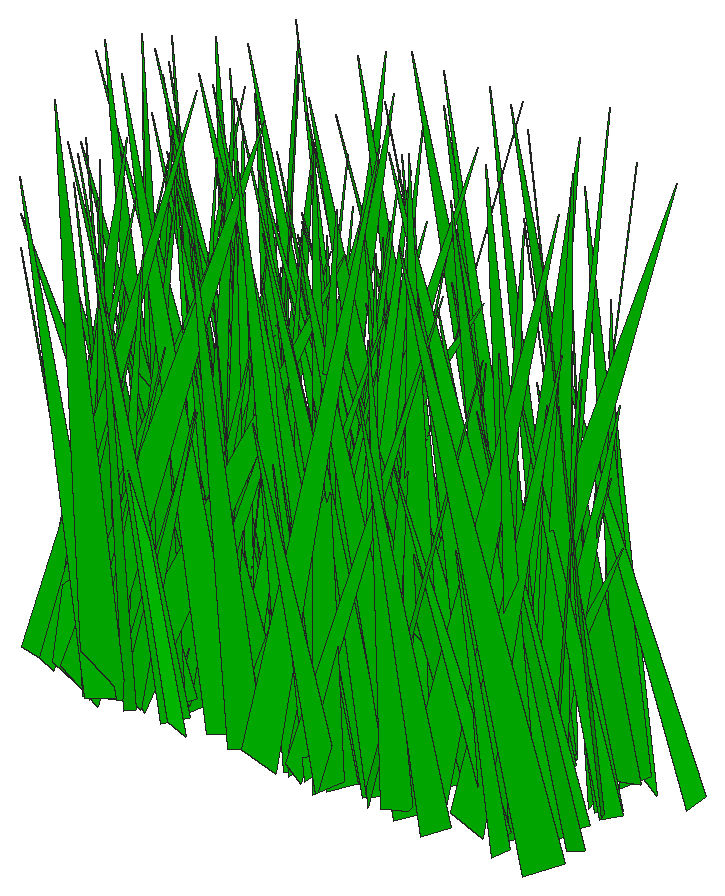
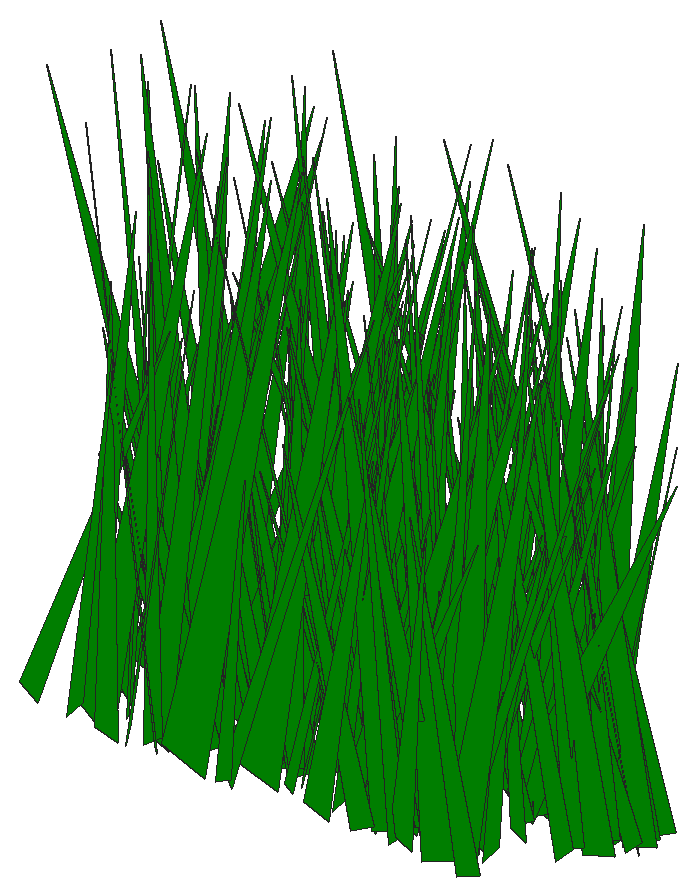
# SketchUp Ruby script. Lengths in inches.
U = 1.inch
M = Sketchup.active_model
def pt(a) = Geom::Point3d.new(a.map { |v| v * U })
def face(e, loops, mat)
  f = e.add_face(loops[0].map { |a| pt(a) })
  loops[1..].each { |l| e.add_face(l.map { |a| pt(a) }).erase! }
  f.material = f.back_material = mat if mat
  f
end
# faces: each face lists its corners as indices into pts; further lists are holes
def faces(e, pts, list, mat = nil) = list.each { |f| face(e, (f[0].is_a?(Array) ? f : [f]).map { |l| l.map { |i| pts[i] } }, mat) }
# xy, xz, yz: faces in a plane at the given z, y or x. An outline is a flat list of corners, or four numbers for a rectangle; further outlines are holes
def ring(l) = l.size == 4 ? [[l[0], l[1]], [l[2], l[1]], [l[2], l[3]], [l[0], l[3]]] : l.each_slice(2).to_a
def flat(e, list, mat, &to3) = list.each { |f| face(e, (f[0].is_a?(Array) ? f : [f]).map { |l| ring(l).map { |u, v| to3.(u, v) } }, mat) }
def xy(e, z, list, mat = nil) = flat(e, list, mat) { |x, y| [x, y, z] }
def xz(e, y, list, mat = nil) = flat(e, list, mat) { |x, z| [x, y, z] }
def yz(e, x, list, mat = nil) = flat(e, list, mat) { |y, z| [x, y, z] }
def lines(e, pts, list) = list.each { |a, b| e.add_line(pt(pts[a]), pt(pts[b])) }
# prism: a flat outline (further loops are holes) pulled along v
def prism(e, loops, v, mat = nil)
  f = face(e, loops, mat); d = Geom::Vector3d.new(v.map { |x| x * U })
  f.pushpull(f.normal.samedirection?(d) ? d.length : -d.length)
end
def box(e, o, s, mat = nil) = prism(e, [[o, [o[0] + s[0], o[1], o[2]], [o[0] + s[0], o[1] + s[1], o[2]], [o[0], o[1] + s[1], o[2]]]], [0, 0, s[2]], mat)
def at(x, y, z, deg = 0) = Geom::Transformation.translation(pt([x, y, z])) * Geom::Transformation.rotation(ORIGIN, Z_AXIS, deg.degrees)
def axes(o, x, y, z) = Geom::Transformation.new([*x, 0, *y, 0, *z, 0, *pt(o).to_a, 1])
def part(name) = M.definitions.add(name)
# library, detail: a bought-in or finely detailed component or shape, given as its bounding box
def library(name, o, s) = part(name).tap { |d| box(d.entities, o, s) }
def detail(e, o, s) = box(e.add_group.entities, o, s)
def put(e, d, t, mat = nil) = e.add_instance(d, t).tap { |i| i.material = mat if mat }
def group(e, t, mat = nil) = e.add_group.tap { |g| g.transformation = t; g.material = mat if mat }.entities
root = M.entities
M.materials.add("[Color G06]").color = [0, 204, 0]
c1 = part("fur_instance\#9")
p = [[0.8125,0,1.79],[0.67,-0.02,1.48],[0,-0.11,0],[0,0.11,0]]
faces(c1.entities,p,[[0,1,2,3]])
put(root,c1,axes([80.09,16.16,4.28],[-3.96504,0.00462,0.61887],[-0.1065,0.52435,-1.97341],[0.40152,0.18466,5.58803]),"[Color G06]")
put(root,c1,axes([81.36,17.7,4.28],[-2.4045,0.50598,0.05745],[3.24631,0.29707,2.94108],[-1.62149,-0.15557,5.80301]),"[Color G06]")
put(root,c1,axes([77.95,17.43,4.28],[1.58448,-0.59409,2.33966],[-4.52208,-0.18675,1.39339],[0.39011,0.24818,6.64912]),"[Color G06]")
put(root,c1,axes([81.13,20.35,4.28],[-5.10358,0.12595,0.06674],[0.89659,0.70004,1.38494],[-0.11823,-0.12831,7.62141]),"[Color G06]")
put(root,c1,axes([78.5,17.36,4.28],[-2.23107,0.3733,1.08265],[2.29187,0.32118,-2.17174],[1.56163,0.06197,4.73401]),"[Color G06]")
put(root,c1,axes([80.28,15.98,4.28],[-2.39441,0.52902,0.87524],[3.82716,0.32155,1.06103],[-0.29682,-0.12147,6.6204]),"[Color G06]")
put(root,c1,axes([79.65,17.76,4.28],[-4.27684,-0.24388,1.66183],[-1.50261,0.60978,1.64164],[1.4273,-0.08881,6.70788]),"[Color G06]")
put(root,c1,axes([77.92,16.99,4.28],[3.84261,0.30678,1.26542],[2.34016,-0.52363,-1.29043],[-0.2839,-0.16391,6.49069]),"[Color G06]")
put(root,c1,axes([78.72,17.62,4.28],[1.63511,0.35667,2.41092],[3.02113,-0.2038,-1.11332],[-0.13155,-0.24709,4.39848]),"[Color G06]")
put(root,c1,axes([78.9,16.41,4.28],[-1.91184,0.4234,1.31875],[2.85671,0.29293,-1.5526],[1.35528,-0.02017,5.13294]),"[Color G06]")
put(root,c1,axes([78.42,17.22,4.28],[3.46241,0.21076,0.30932],[1.42342,-0.47208,1.36022],[-0.54874,0.10528,5.48009]),"[Color G06]")
put(root,c1,axes([78.36,16.45,4.28],[2.42093,-0.21005,0.71566],[-1.58046,-0.31995,1.15486],[0.02258,0.12672,4.10204]),"[Color G06]")
put(root,c1,axes([78.46,18.35,4.28],[0.43266,0.63211,0.99472],[4.49647,-0.0407,-1.39792],[0.8791,-0.10294,6.66058]),"[Color G06]")
put(root,c1,axes([78.11,17.37,4.28],[4.86594,0.18567,0.54154],[1.17861,-0.65553,2.16249],[-0.71768,0.18233,7.2231]),"[Color G06]")
put(root,c1,axes([79.97,17.38,4.28],[-4.23289,-0.34339,0.66218],[-2.11478,0.5559,2.9186],[1.33719,-0.20785,6.71195]),"[Color G06]")
put(root,c1,axes([81.48,17.78,4.28],[-4.50555,-0.20228,0.60661],[-1.50622,0.60311,-1.8868],[-0.01596,0.1849,6.81801]),"[Color G06]")
put(root,c1,axes([80.9,20.61,4.28],[0.2752,-0.65623,1.88496],[-4.66441,-0.08636,-1.93271],[-1.40715,0.15794,6.77517]),"[Color G06]")
put(root,c1,axes([79.14,18.41,4.28],[3.6223,0.36259,2.56895],[2.99852,-0.5057,-1.24506],[-0.85112,-0.23845,6.54687]),"[Color G06]")
put(root,c1,axes([79.79,16.81,4.28],[-3.23329,-0.49254,1.52623],[-3.33124,0.47268,1.75922],[1.55612,-0.01151,6.93722]),"[Color G06]")
put(root,c1,axes([80.375,16.03,4.28],[0.81309,-0.78469,0.50058],[-5.56406,-0.11929,-1.29318],[-0.90518,0.0284,8.3987]),"[Color G06]")
put(root,c1,axes([81.125,19.6875,4.28],[-0.21231,0.4211,1.68724],[3.02032,-0.0292,1.68604],[-1.12756,-0.1575,4.19858]),"[Color G06]")
put(root,c1,axes([81.89,16.99,4.28],[-2.15082,0.47994,0.40651],[3.29774,0.27236,2.03593],[-1.02201,-0.13119,5.71389]),"[Color G06]")
put(root,c1,axes([80.46,19.91,4.28],[-4.83651,-0.45011,1.24887],[-2.8033,0.66008,3.07866],[1.80518,-0.18089,8.12692]),"[Color G06]")
put(root,c1,axes([81.21,17.43,4.28],[0.82147,0.73645,2.48814],[5.30748,-0.17164,1.92187],[-1.57919,-0.19378,7.7535]),"[Color G06]")
put(root,c1,axes([77.89,16.61,4.28],[5.38802,-0.39803,0.24516],[-2.84975,-0.7437,1.1956],[0.23092,0.10922,9.03424]),"[Color G06]")
put(root,c1,axes([80.7,17.61,4.28],[-4.16965,0.39593,1.84315],[2.72244,0.60634,-1.20494],[1.47337,0.00011,7.44256]),"[Color G06]")
put(root,c1,axes([81.95,19,4.28],[-2.47231,0.30424,0.98661],[2.19111,0.27974,2.35509],[-0.62856,-0.22153,4.329]),"[Color G06]")
put(root,c1,axes([78.05,17.54,4.28],[4.01317,0.37829,0.17792],[2.59468,-0.52549,-2.38462],[0.80068,-0.19316,6.83579]),"[Color G06]")
put(root,c1,axes([79.08,18.86,4.28],[5.07893,-0.20615,1.62963],[-1.70837,-0.69439,1.80264],[-0.67517,0.20626,7.6976]),"[Color G06]")
put(root,c1,axes([81.15,15.97,4.28],[3.31982,0.29513,2.99147],[2.00912,-0.5384,1.12136],[-2.10928,-0.04832,5.77642]),"[Color G06]")
put(root,c1,axes([82.82,17.6,4.28],[-2.6484,-0.58234,1.01179],[-4.0563,0.31788,-2.69933],[-1.20194,0.21035,6.88023]),"[Color G06]")
put(root,c1,axes([80.11,16.8,4.28],[3.64205,-0.35592,0.44862],[-2.36631,-0.49274,-1.99603],[-1.00267,-0.12994,6.34016]),"[Color G06]")
put(root,c1,axes([81.54,19.76,4.28],[0.99429,0.79231,0.0814],[5.53838,-0.13686,1.91316],[-1.27012,0.02348,8.40609]),"[Color G06]")
put(root,c1,axes([79.84,16.05,4.28],[3.50765,-0.04486,0.99817],[-0.56639,-0.45277,2.10829],[-0.47827,0.20717,4.82385]),"[Color G06]")
put(root,c1,axes([82.6,17.38,4.28],[-3.57372,-0.17571,0.20364],[-1.24049,0.47327,-1.71721],[-0.25986,0.15722,5.39686]),"[Color G06]")
put(root,c1,axes([82.54,15.93,4.28],[-4.81615,0.25556,0.10319],[1.78872,0.66051,-1.43588],[0.40512,0.12186,7.56662]),"[Color G06]")
put(root,c1,axes([80.23,16.99,4.28],[3.20722,0.40339,2.50922],[3.29254,-0.43784,-1.31478],[-0.58841,-0.25125,6.3199]),"[Color G06]")
put(root,c1,axes([78.59,16.93,4.28],[2.98606,-0.61165,0.26624],[-4.16026,-0.3847,2.70231],[1.40121,0.16127,7.45594]),"[Color G06]")
put(root,c1,axes([81.77,16.75,4.28],[4.04095,0.57837,2.58795],[3.68795,-0.61227,2.85567],[-2.5691,0.0308,8.16993]),"[Color G06]")
put(root,c1,axes([80.54,18.77,4.28],[4.36803,-0.24739,1.48073],[-1.54639,-0.61719,-1.65582],[-1.31822,-0.09573,6.84895]),"[Color G06]")
put(root,c1,axes([82.59,18.78,4.28],[-1.58143,0.40161,0.24801],[2.74135,0.20099,1.65805],[-0.89849,-0.09364,4.6223]),"[Color G06]")
put(root,c1,axes([82.26,16.23,4.28],[0.70188,-0.54769,1.43807],[-3.75426,-0.13886,-1.9821],[-1.50258,0.09111,5.6241]),"[Color G06]")
put(root,c1,axes([80.24,21.03,4.28],[1.16188,-0.42472,0.47893],[-3.01179,-0.14979,1.06163],[0.5554,0.07622,4.75501]),"[Color G06]")
put(root,c1,axes([81.04,19.32,4.28],[2.43605,-0.25594,0.32134],[-1.63588,-0.32174,-1.73621],[-0.85956,-0.11302,4.21501]),"[Color G06]")
put(root,c1,axes([83.5,19.28,4.28],[-4.86937,0.36862,1.36795],[2.79614,0.63358,2.62044],[-0.08479,-0.27555,7.85534]),"[Color G06]")
put(root,c1,axes([81.9,20.03,4.28],[-4.57528,0.18823,3.13164],[1.9138,0.65659,1.71217],[1.59683,-0.24761,6.92083]),"[Color G06]")
put(root,c1,axes([83.37,18.5,4.28],[-4.60442,0.28891,0.86362],[2.1486,0.62669,1.50444],[0.10062,-0.16124,7.39477]),"[Color G06]")
put(root,c1,axes([80.6,16.57,4.28],[0.32697,-0.38482,1.37835],[-2.73268,0.00383,1.57089],[0.99929,0.13639,3.8448]),"[Color G06]")
put(root,c1,axes([82.48,17.54,4.28],[-0.30271,0.39217,0.95163],[2.805,0.01935,1.07699],[-0.6685,-0.09639,4.0881]),"[Color G06]")
put(root,c1,axes([82.28,19.53,4.28],[0.708,-0.5248,0.93803],[-3.7172,-0.11495,-1.12057],[-0.86046,0.06476,5.61274]),"[Color G06]")
put(root,c1,axes([82.01,19.58,4.28],[-2.39476,-0.4155,0.18423],[-2.85308,0.32562,1.52115],[0.86817,-0.07604,5.50717]),"[Color G06]")
put(root,c1,axes([80.94,16.3125,4.28],[1.54694,0.33616,0.96474],[2.47753,-0.19414,-1.10306],[0.29989,-0.13017,4.13641]),"[Color G06]")
put(root,c1,axes([83.54,16.49,4.28],[-2.62366,0.70015,1.24289],[5.05123,0.3423,1.66728],[-0.62171,-0.17358,8.30114]),"[Color G06]")
put(root,c1,axes([83.1,19.95,4.28],[0.71881,-0.58378,0.80663],[-3.92306,-0.12057,-2.21494],[-1.55795,0.03426,5.94958]),"[Color G06]")
put(root,c1,axes([82.52,20.74,4.28],[0.67687,0.44536,0.3364],[3.07735,-0.09935,1.27806],[-0.88357,-0.00485,4.70898]),"[Color G06]")
put(root,c1,axes([80.77,18.22,4.28],[2.3137,0.35161,0.89932],[2.56104,-0.29262,-1.57519],[0.40143,-0.15971,4.86608]),"[Color G06]")
put(root,c1,axes([81.23,20.91,4.28],[-0.73264,-0.68843,0.33457],[-4.769,0.10676,1.9084],[1.29609,0.00369,7.21113]),"[Color G06]")
put(root,c1,axes([81.78,19.58,4.28],[3.83466,-0.10946,2.37796],[-1.12493,-0.5586,1.09833],[-1.37193,0.15207,5.74599]),"[Color G06]")
put(root,c1,axes([83.74,17.68,4.28],[-5.72432,-0.07873,1.63527],[-0.93594,0.74967,-3.1724],[0.79994,0.31376,7.99019]),"[Color G06]")
put(root,c1,axes([79.58,16.12,4.28],[3.16824,0.74272,0.60226],[5.15125,-0.40757,-2.7925],[1.41278,-0.17952,8.83135]),"[Color G06]")
put(root,c1,axes([83.78,20.46,4.28],[-1.65602,-0.40717,0.43226],[-2.72838,0.19664,-2.07052],[-1.07954,0.12761,4.56983]),"[Color G06]")
put(root,c1,axes([84.27,19.66,4.28],[-3.87879,0.52171,0.42569],[3.70429,0.52334,1.71482],[-0.59736,-0.14226,7.86975]),"[Color G06]")
put(root,c1,axes([83.77,17.71,4.28],[-0.12418,-0.69923,0.11328],[-4.71267,0.01266,-2.56608],[-1.71484,0.01586,7.04383]),"[Color G06]")
put(root,c1,axes([82.5,18.28,4.28],[-3.40951,0.52314,1.3132],[3.59675,0.49079,-1.60056],[1.38195,0.01331,7.40564]),"[Color G06]")
put(root,c1,axes([83.08,16.58,4.28],[-4.76756,0.23054,1.68564],[1.47211,0.67923,-1.37104],[1.3558,0.07317,7.41606]),"[Color G06]")
put(root,c1,axes([82.35,17.15,4.28],[4.03013,0.64486,0.15163],[4.28978,-0.52808,3.3066],[-1.73031,0.19277,8.55088]),"[Color G06]")
put(root,c1,axes([82.41,19.34,4.28],[4.96519,0.45977,1.55514],[2.76899,-0.68085,3.37523],[-2.07035,0.19203,8.24378]),"[Color G06]")
put(root,c1,axes([81.57,17.21,4.28],[-0.53189,-0.41062,2.41143],[-3.05598,0.15358,1.49841],[1.3911,0.18038,4.21372]),"[Color G06]")
put(root,c1,axes([81.42,20.64,4.28],[0.81439,0.59826,0.36984],[4.18237,-0.10227,-1.5681],[0.98764,-0.06024,6.33544]),"[Color G06]")
put(root,c1,axes([83.79,19.01,4.28],[-4.3787,-0.31758,0.36115],[-2.15416,0.5958,1.84404],[0.77758,-0.13777,7.14234]),"[Color G06]")
put(root,c1,axes([82.88,17.54,4.28],[1.86528,0.58077,0.34705],[4.04047,-0.26037,1.54429],[-1.03668,0.03018,6.64334]),"[Color G06]")
put(root,c1,axes([85.39,18.63,4.28],[-4.17033,0.42514,0.08923],[2.86207,0.54084,2.7787],[-1.05236,-0.21389,7.20354]),"[Color G06]")
put(root,c1,axes([83.98,19.09,4.28],[1.74604,0.75305,0.44387],[4.99882,-0.24131,3.10552],[-2.06482,0.05259,7.89364]),"[Color G06]")
put(root,c1,axes([82.45,18.3,4.28],[3.80681,0.12833,1.46285],[0.57715,-0.52655,1.95156],[-1.21321,0.15219,5.51854]),"[Color G06]")
put(root,c1,axes([83.26,19.1875,4.28],[1.87152,-0.72948,0.52679],[-5.11595,-0.26549,-1.63416],[-1.14797,-0.00609,8.14147]),"[Color G06]")
put(root,c1,axes([82.64,20.72,4.28],[3.48071,-0.19732,2.6462],[-1.99959,-0.48037,1.76035],[-1.06715,0.25649,5.33259]),"[Color G06]")
put(root,c1,axes([83.52,17.32,4.28],[-3.46008,-0.14982,1.3927],[-0.8941,0.49495,1.15466],[1.10601,-0.06859,5.29038]),"[Color G06]")
put(root,c1,axes([82.79,18.76,4.28],[5.25675,0.11325,2.77653],[0.2932,-0.75477,2.29663],[-2.0062,0.18644,7.61086]),"[Color G06]")
put(root,c1,axes([82.74,17.22,4.28],[3.57711,0.39826,0.4126],[2.65145,-0.48231,2.13218],[-1.09673,0.13292,6.5005]),"[Color G06]")
put(root,c1,axes([84.54,20.16,4.28],[-2.0182,-0.34557,0.81583],[-2.49557,0.25267,-1.49552],[-0.45975,0.14544,4.5365]),"[Color G06]")
put(root,c1,axes([84.72,20.3,4.28],[-5.59106,0.18018,1.37785],[1.1167,0.78103,-1.61102],[1.12807,0.1199,8.42385]),"[Color G06]")
put(root,c1,axes([83.03,19.55,4.28],[4.8492,0.30832,1.14131],[1.64095,-0.62303,3.76062],[-1.66705,0.28357,7.02165]),"[Color G06]")
put(root,c1,axes([84.42,16.38,4.28],[0.62086,-0.43252,2.31952],[-3.23287,-0.15179,-1.31847],[-1.25604,0.17689,4.5401]),"[Color G06]")
put(root,c1,axes([82.96,17.78,4.28],[-1.29724,0.38675,0.56168],[2.50069,0.1861,-1.81916],[1.25691,0.02889,4.19902]),"[Color G06]")
put(root,c1,axes([80.54,16.74,4.28],[3.12174,0.6349,0.68513],[4.10065,-0.35378,-4.07492],[2.03102,-0.26158,7.17424]),"[Color G06]")
put(root,c1,axes([81.65,17.25,4.28],[4.85334,-0.136,0.46895],[-1.02292,-0.63151,2.6097],[0.05684,0.24726,6.92315]),"[Color G06]")
put(root,c1,axes([84.31,16.22,4.28],[1.00307,-0.64992,0.68496],[-4.54914,-0.15074,-1.54979],[-1.11252,0.03042,6.9547]),"[Color G06]")
put(root,c1,axes([85.4,18.62,4.28],[-2.01536,0.31367,0.15616],[2.11287,0.25664,1.69171],[-0.7789,-0.11545,4.18492]),"[Color G06]")
put(root,c1,axes([82.99,20.49,4.28],[2.4073,-0.65825,3.0239],[-5.13582,-0.30887,1.40913],[-0.00544,0.31126,7.7932]),"[Color G06]")
put(root,c1,axes([85.91,19.02,4.28],[-4.65742,0.48174,1.27383],[3.55823,0.62987,1.69646],[-0.01219,-0.19793,8.4991]),"[Color G06]")
put(root,c1,axes([82.9,20.02,4.28],[2.00621,0.71297,1.16865],[5.15535,-0.26615,-1.1162],[0.41928,-0.13898,8.13261]),"[Color G06]")
put(root,c1,axes([84.96,20.86,4.28],[0.45118,-0.46763,1.51795],[-3.33315,-0.10132,-1.37248],[-1.08056,0.11727,4.86741]),"[Color G06]")
put(root,c1,axes([86.17,20.4,4.28],[-5.1128,0.07158,0.87637],[0.61443,0.70404,1.4015],[0.47936,-0.13898,7.5509]),"[Color G06]")
put(root,c1,axes([84.625,19.17,4.28],[3.05046,-0.38118,1.79135],[-2.60789,-0.45662,-1.24176],[-1.45179,0.01932,5.99456]),"[Color G06]")
put(root,c1,axes([82.97,20.14,4.28],[2.49245,0.55072,0.25683],[3.89607,-0.33743,-1.34059],[0.66905,-0.08669,6.84984]),"[Color G06]")
put(root,c1,axes([84.35,18.4375,4.28],[-2.55369,0.3782,1.91782],[2.63333,0.39513,-1.11857],[1.43803,-0.05195,5.45406]),"[Color G06]")
put(root,c1,axes([83.95,17.6,4.28],[4.422,-0.37219,0.66523],[-2.41219,-0.59609,-2.49382],[-1.22607,-0.16959,7.30565]),"[Color G06]")
put(root,c1,axes([83.61,20.82,4.28],[1.58458,-0.42734,0.73945],[-3.02989,-0.19606,1.48741],[0.67549,0.12307,4.93712]),"[Color G06]")
put(root,c1,axes([86.14,19.89,4.28],[-4.23088,-0.12454,0.38843],[-0.74805,0.55589,2.27377],[0.55282,-0.20094,6.04951]),"[Color G06]")
put(root,c1,axes([85.99,16.2,4.28],[1.45315,-0.6407,3.20792],[-4.78351,-0.27656,-1.50505],[-1.68401,0.23272,7.04331]),"[Color G06]")
put(root,c1,axes([84.42,19.73,4.28],[-1.57082,0.417,0.89836],[2.68422,0.23376,-1.9806],[1.44873,0.01903,4.64375]),"[Color G06]")
put(root,c1,axes([86.98,16.59,4.28],[-5.59106,0.29296,1.64826],[2.32967,0.75248,2.28801],[0.45027,-0.2555,8.62853]),"[Color G06]")
put(root,c1,axes([87.49,18.58,4.28],[-4.97977,0.22547,0.49486],[1.63188,0.65069,2.62492],[-0.24679,-0.24683,7.37172]),"[Color G06]")
put(root,c1,axes([87.625,20.89,4.28],[-4.92815,-0.25982,0.21604],[-1.84957,0.66994,-1.68903],[-0.26775,0.15442,7.69107]),"[Color G06]")
put(root,c1,axes([85.86,16.11,4.28],[1.88508,0.34433,0.36024],[2.14355,-0.24729,2.09744],[-1.24931,0.09527,4.14231]),"[Color G06]")
put(root,c1,axes([81.9,18.91,4.28],[3.91029,0.55594,0.32528],[3.26459,-0.42071,-5.06229],[2.29882,-0.3482,6.63574]),"[Color G06]")
put(root,c1,axes([85.79,17.95,4.28],[3.43986,-0.09494,2.53886],[-0.38777,-0.53069,-1.10605],[-1.78851,-0.06753,5.12281]),"[Color G06]")
put(root,c1,axes([87.06,20.42,4.28],[-2.53338,0.67432,2.23538],[5.0391,0.31393,1.87795],[-0.4786,-0.26409,7.94008]),"[Color G06]")
put(root,c1,axes([87.31,19.15,4.28],[-0.42874,-0.80659,1.02932],[-5.61203,0.03139,-2.39625],[-1.56122,0.10868,8.33099]),"[Color G06]")
put(root,c1,axes([87.15,16.17,4.28],[0.53643,0.63029,1.01283],[4.22194,-0.10478,2.49538],[-1.75056,-0.05956,6.32862]),"[Color G06]")
put(root,c1,axes([87.84,16.9,4.28],[-6.10604,0.02884,0.85155],[0.34118,0.8283,2.24265],[0.50098,-0.21264,8.85148]),"[Color G06]")
put(root,c1,axes([86.29,16.06,4.28],[-2.48734,0.1156,1.40749],[1.09528,0.34229,1.09425],[0.61191,-0.14279,3.76266]),"[Color G06]")
put(root,c1,axes([87.76,17.52,4.28],[-5.12712,-0.21332,0.80868],[-1.59379,0.70899,-1.08737],[0.3046,0.11909,7.9224]),"[Color G06]")
put(root,c1,axes([83.875,16.57,4.28],[4.63048,-0.19273,0.29295],[-1.37833,-0.61626,2.09195],[0.22088,0.19466,6.91269]),"[Color G06]")
put(root,c1,axes([86.85,16.01,4.28],[1.51599,-0.46498,0.42742],[-2.8969,-0.20424,-2.57208],[-1.67589,-0.06758,4.83267]),"[Color G06]")
put(root,c1,axes([84.75,17.06,4.28],[3.05855,-0.32381,0.63285],[-2.35643,-0.41325,1.14906],[0.1373,0.12089,5.62325]),"[Color G06]")
put(root,c1,axes([84.78,19.65,4.28],[4.27,0.18114,1.03188],[1.41037,-0.58811,-1.17726],[-0.41818,-0.13392,6.56588]),"[Color G06]")
put(root,c1,axes([84.9,19.52,4.28],[3.19367,-0.01663,0.09811],[-0.1358,-0.40469,1.99257],[-0.00985,0.18613,4.34105]),"[Color G06]")
put(root,c1,axes([87.59,16.91,4.28],[-0.83097,-0.53377,1.30442],[-3.79131,0.07678,-1.78562],[-1.01984,0.14948,5.57528]),"[Color G06]")
put(root,c1,axes([85.5,17.74,4.28],[-2.07005,0.51137,3.63729],[3.95636,0.38051,-1.11571],[1.92821,-0.23175,6.19408]),"[Color G06]")
put(root,c1,axes([86.91,15.95,4.28],[3.60081,0.68369,1.10858],[4.44381,-0.50163,3.29712],[-2.2004,0.10575,8.47281]),"[Color G06]")
put(root,c1,axes([86.79,19.63,4.28],[-2.52599,0.56975,0.28934],[4.02625,0.35192,-1.09066],[0.72183,0.03086,7.09605]),"[Color G06]")
put(root,c1,axes([85.86,16.71,4.28],[-0.16651,-0.77025,0.37189],[-5.48327,0.02747,1.05211],[0.71178,0.03144,8.19199]),"[Color G06]")
put(root,c1,axes([88.01,16.48,4.28],[-0.10922,-0.70069,1.17539],[-4.79681,-0.02227,-2.52055],[-1.69049,0.10845,7.0762]),"[Color G06]")
put(root,c1,axes([85.45,17.56,4.28],[5.10483,-0.15196,2.17176],[-1.39846,-0.71455,1.59925],[-1.15902,0.19288,7.63577]),"[Color G06]")
put(root,c1,axes([87.38,18.91,4.28],[-0.91204,0.48361,0.66321],[3.44777,0.11378,1.06039],[-0.58077,-0.08402,5.25357]),"[Color G06]")
put(root,c1,axes([87.24,18.85,4.28],[0.37583,-0.59118,2.07254],[-4.34634,-0.09216,-1.25945],[-1.00285,0.17789,6.23518]),"[Color G06]")
put(root,c1,axes([87.43,16.64,4.28],[1.26493,0.69912,1.94954],[4.92497,-0.22037,1.94008],[-1.60696,-0.12505,7.48051]),"[Color G06]")
put(root,c1,axes([84.4375,20.14,4.28],[6.16569,0.14954,0.17446],[1.01689,-0.83727,2.16276],[-0.35989,0.19612,9.09993]),"[Color G06]")
put(root,c1,axes([84.91,15.94,4.28],[4.73646,-0.5121,1.81169],[-3.86207,-0.64023,1.76522],[-0.20082,0.23433,8.78189]),"[Color G06]")
put(root,c1,axes([86.79,17.86,4.28],[-2.71326,0.55494,0.64136],[3.84746,0.38152,-1.56369],[1.10384,0.03425,7.02679]),"[Color G06]")
put(root,c1,axes([87.5625,19.49,4.28],[-4.43128,0.37129,0.9482],[2.521,0.61919,-1.53568],[1.06614,0.07908,7.57235]),"[Color G06]")
put(root,c1,axes([89,17.68,4.28],[-3.68283,0.48213,0.36531],[3.38434,0.48945,2.00717],[-0.74849,-0.15918,7.27812]),"[Color G06]")
put(root,c1,axes([84.39,17.92,4.28],[5.50058,-0.39536,1.59384],[-3.01535,-0.68523,3.7194],[0.28912,0.37539,8.46804]),"[Color G06]")
put(root,c1,axes([86.08,17.34,4.28],[-3.97135,0.52358,2.54327],[3.09745,0.59642,-3.30074],[2.72016,0.08526,7.47167]),"[Color G06]")
put(root,c1,axes([87,18.8125,4.28],[3.69339,0.00535,2.62755],[-0.67953,-0.52164,2.25569],[-1.62188,0.23075,5.03845]),"[Color G06]")
put(root,c1,axes([87.6,17.4,4.28],[1.20833,0.5891,0.61933],[4.09101,-0.17764,1.58156],[-1.13252,-0.01316,6.37389]),"[Color G06]")
put(root,c1,axes([88.03,16.41,4.28],[0.23182,-0.47401,1.30535],[-3.33461,-0.06781,-1.5059],[-1.09451,0.10621,4.86445]),"[Color G06]")
put(root,c1,axes([86.34,20.17,4.28],[3.39193,-0.02269,0.69241],[-0.05855,-0.46639,-1.11502],[-0.48753,-0.10186,4.95132]),"[Color G06]")
put(root,c1,axes([87.37,16.86,4.28],[-3.90598,0.37922,1.54539],[2.38324,0.55549,-2.20315],[1.66879,0.0943,6.76354]),"[Color G06]")
put(root,c1,axes([86.14,17.85,4.28],[5.26577,-0.4469,0.99376],[-3.09451,-0.73697,-1.44461],[-1.06639,-0.0682,9.09913]),"[Color G06]")
put(root,c1,axes([88.94,20.92,4.28],[-1.02421,-0.85485,0.6874],[-6.00757,0.12538,-2.08308],[-1.3046,0.09376,9.0527]),"[Color G06]")
put(root,c1,axes([89.17,16.14,4.28],[-0.31364,0.68265,1.91741],[4.72834,-0.02436,2.72414],[-1.80398,-0.18255,6.80678]),"[Color G06]")
put(root,c1,axes([87.6,21.08,4.28],[-1.95022,-0.32992,0.18694],[-2.26555,0.26629,1.19314],[0.69334,-0.05787,4.4245]),"[Color G06]")
put(root,c1,axes([86.25,19.54,4.28],[0.17932,-0.479,0.19205],[-3.20619,-0.01684,1.86315],[1.23954,0.02575,4.79144]),"[Color G06]")
put(root,c1,axes([89.52,18.46,4.28],[-2.25287,0.49977,0.34091],[3.44194,0.28977,2.00908],[-1.02462,-0.12544,5.9994]),"[Color G06]")
put(root,c1,axes([90.48,17.21,4.28],[-4.02947,-0.48782,0.63891],[-3.31639,0.49419,-3.37496],[-1.19267,0.27395,7.226]),"[Color G06]")
put(root,c1,axes([85.88,15.98,4.28],[5.00397,-0.18864,0.53122],[-1.39783,-0.66795,2.16456],[0.0494,0.20783,7.43874]),"[Color G06]")
put(root,c1,axes([87.81,16.74,4.28],[2.82918,0.47306,0.07354],[3.23993,-0.37936,1.90056],[-1.00683,0.10853,6.32253]),"[Color G06]")
put(root,c1,axes([87.21,19.69,4.28],[0.87377,-0.40079,0.1149],[-2.79226,-0.11561,1.10466],[0.68572,0.03993,4.3518]),"[Color G06]")
put(root,c1,axes([89.71,20.04,4.28],[-1.34759,-0.70429,3.01603],[-5.36345,0.12397,-2.02766],[-0.9027,0.31485,7.54495]),"[Color G06]")
put(root,c1,axes([88.48,17.42,4.28],[2.36068,-0.75604,1.15423],[-5.37158,-0.3425,-1.23116],[-1.06697,0.05153,8.75188]),"[Color G06]")
put(root,c1,axes([88.76,16.13,4.28],[1.1698,-0.58371,0.85569],[-4.1427,-0.17474,-1.04221],[-0.8295,0.0495,6.41178]),"[Color G06]")
put(root,c1,axes([88.56,17.14,4.28],[-1.98046,0.39942,0.37759],[2.7556,0.27585,-1.2361],[0.82164,0.03761,5.05573]),"[Color G06]")
put(root,c1,axes([90.58,18.34,4.28],[-6.08332,-0.03394,0.98566],[-0.13101,0.84181,1.52411],[0.69066,-0.13929,8.9707]),"[Color G06]")
put(root,c1,axes([90.16,19.59,4.28],[-5.24759,0.36003,2.32513],[2.88517,0.72605,1.63037],[0.87307,-0.23533,8.58743]),"[Color G06]")
put(root,c1,axes([90.04,20.54,4.28],[-4.18707,-0.49195,2.49978],[-3.84109,0.58032,-1.2521],[0.69958,0.24193,8.08668]),"[Color G06]")
put(root,c1,axes([90.18,17.65,4.28],[-0.21903,0.65624,0.83585],[4.57412,0.00885,1.87953],[-1.23997,-0.08328,6.78573]),"[Color G06]")
put(root,c1,axes([90.39,19.93,4.28],[-0.35227,-0.63209,1.87942],[-4.4844,-0.00798,-2.18587],[-1.42063,0.18193,6.43393]),"[Color G06]")
put(root,c1,axes([90.07,15.89,4.28],[1.06754,-0.56471,0.39331],[-3.76579,-0.15199,-2.23678],[-1.51267,-0.02016,5.84604]),"[Color G06]")
put(root,c1,axes([90.53,19.33,4.28],[-2.70662,-0.45145,1.2715],[-3.33448,0.35025,-1.56959],[-0.29341,0.18397,6.10839]),"[Color G06]")
put(root,c1,axes([88.32,19.01,4.28],[2.44007,0.16849,0.77671],[1.3153,-0.31248,-1.44313],[0.00077,-0.15291,3.80501]),"[Color G06]")
put(root,c1,axes([87.89,18.73,4.28],[0.1059,0.42996,0.66405],[2.70519,0.01805,-2.30617],[1.54482,-0.06108,3.99289]),"[Color G06]")
put(root,c1,axes([89,17.58,4.28],[3.78851,0.27402,0.88227],[1.56973,-0.49838,2.72532],[-1.32138,0.1936,5.76708]),"[Color G06]")
put(root,c1,axes([90.82,18.28,4.28],[1.42943,0.55389,1.91384],[3.50963,-0.26167,2.84428],[-2.25826,-0.05607,5.6318]),"[Color G06]")
put(root,c1,axes([90.74,20.73,4.28],[-4.78335,0.06856,1.10733],[0.21878,0.63867,-2.43137],[0.86186,0.21838,6.76295]),"[Color G06]")
put(root,c1,axes([90.44,19.01,4.28],[-4.76305,0.02574,1.8472],[-0.18194,0.65761,-2.10078],[1.23633,0.19596,6.80729]),"[Color G06]")
put(root,c1,axes([87.85,16.2,4.28],[4.76341,0.06958,0.48958],[0.5718,-0.63734,-2.02147],[-0.17129,-0.19258,6.86687]),"[Color G06]")
put(root,c1,axes([91.41,16.625,4.28],[-2.58127,0.30072,0.34692],[2.08275,0.32959,1.79549],[-0.60569,-0.14825,4.69556]),"[Color G06]")
put(root,c1,axes([92.4,17.34,4.28],[-3.53131,0.67533,0.94366],[4.74002,0.44773,2.81447],[-1.17684,-0.22311,8.50439]),"[Color G06]")
put(root,c1,axes([90.09,20.625,4.28],[-3.74035,0.31437,2.03442],[2.08407,0.55491,-1.2915],[1.61001,0.01205,6.39811]),"[Color G06]")
put(root,c1,axes([90.86,17.83,4.28],[1.61652,-0.75823,1.0183],[-5.25574,-0.24256,-2.11097],[-1.55164,0.03167,8.21123]),"[Color G06]")
put(root,c1,axes([88.77,20.1,4.28],[1.34435,0.4263,1.43993],[3.07181,-0.12973,-1.99407],[0.91561,-0.19069,4.57577]),"[Color G06]")
put(root,c1,axes([89.46,20.12,4.28],[3.23114,0.48853,3.59386],[4.18994,-0.4364,-1.60008],[-0.70712,-0.35355,6.94093]),"[Color G06]")
put(root,c1,axes([89.65,18.01,4.28],[2.83601,0.08828,1.28409],[0.88762,-0.38397,-1.34665],[-0.59251,-0.15269,4.12889]),"[Color G06]")
put(root,c1,axes([91.15,18.76,4.28],[-3.15501,0.02784,0.63326],[0.06696,0.42501,-1.40155],[0.46359,0.12811,4.51216]),"[Color G06]")
put(root,c1,axes([90.81,18.41,4.28],[1.26556,-0.79316,1.20843],[-5.64443,-0.19318,-1.36133],[-1.07107,0.08085,8.60193]),"[Color G06]")
put(root,c1,axes([91.96,20.34,4.28],[1.98652,0.57746,5.60127],[4.93164,-0.44172,1.32438],[-2.62169,-0.39336,6.73551]),"[Color G06]")
put(root,c1,axes([89.97,18.88,4.28],[2.99875,-0.32448,0.42471],[-2.24516,-0.41604,-1.10396],[-0.67431,-0.05777,5.56446]),"[Color G06]")
put(root,c1,axes([89.42,19.4,4.28],[1.91328,-0.81008,1.22455],[-5.85043,-0.25448,1.07948],[0.43763,0.13955,9.07721]),"[Color G06]")
put(root,c1,axes([90.57,17.82,4.28],[-1.13061,0.40535,0.00019],[2.81093,0.15246,-1.18755],[0.74058,0.04015,4.50774]),"[Color G06]")
put(root,c1,axes([90.18,19.84,4.28],[2.96433,0.12084,0.49023],[0.67592,-0.38687,1.82548],[-0.63381,0.15261,4.23953]),"[Color G06]")
put(root,c1,axes([92.47,17.97,4.28],[-1.87718,0.48877,0.52227],[3.38903,0.23555,1.88609],[-0.9603,-0.12414,5.63532]),"[Color G06]")
put(root,c1,axes([90.68,18.29,4.28],[-2.1848,0.22249,1.43832],[1.40615,0.33256,-1.13836],[1.22252,0.0151,3.87981]),"[Color G06]")
put(root,c1,axes([89.79,20.89,4.28],[5.51299,0.0155,1.86573],[0.34877,-0.77322,-1.56412],[-1.20377,-0.15304,8.09145]),"[Color G06]")
put(root,c1,axes([89.81,19.77,4.28],[2.65467,0.20122,0.6524],[1.5056,-0.3475,-1.37238],[0.07771,-0.14136,4.30231]),"[Color G06]")
put(root,c1,axes([89.47,19.81,4.28],[1.2395,-0.33858,0.07067],[-2.16131,-0.15042,1.89007],[1.10747,0.08539,3.60951]),"[Color G06]")
put(root,c1,axes([90.39,17.58,4.28],[-3.2234,-0.59966,2.27921],[-4.02957,0.49627,2.26924],[2.14027,0.03122,7.70504]),"[Color G06]")
put(root,c1,axes([91.3,20.05,4.28],[-4.57992,-0.12872,2.49477],[-0.69618,0.67646,1.15457],[1.77587,-0.06678,6.88656]),"[Color G06]")
put(root,c1,axes([89.05,16.76,4.28],[3.83733,-0.63723,1.46452],[-4.6496,-0.50261,2.09128],[0.47334,0.22888,8.66979]),"[Color G06]")
put(root,c1,axes([90.22,19.64,4.28],[5.77692,-0.12874,2.79412],[-1.26559,-0.82676,1.46896],[-1.65702,0.18264,8.61931]),"[Color G06]")
put(root,c1,axes([91.13,21.07,4.28],[2.83387,-0.41862,1.48606],[-2.91357,-0.418,-1.11575],[-1.22967,0.02566,6.06838]),"[Color G06]")
put(root,c1,axes([92.16,20.5,4.28],[2.43736,0.68492,1.13955],[4.45543,-0.35354,3.12376],[-2.20358,0.04275,7.5764]),"[Color G06]")
put(root,c1,axes([93.07,16.05,4.28],[0.35267,-0.81401,0.79892],[-5.41604,-0.07381,-3.29905],[-2.24237,0.05026,8.09391]),"[Color G06]")
put(root,c1,axes([90.77,19.16,4.28],[3.84353,-0.59236,1.47919],[-4.19545,-0.55239,-1.06047],[-1.19285,0.03418,8.49603]),"[Color G06]")
put(root,c1,axes([90.375,19.37,4.28],[-0.87799,0.54168,0.17586],[3.61433,0.11999,-2.15055],[1.42831,0.02933,5.55009]),"[Color G06]")
put(root,c1,axes([91.84,16.04,4.28],[1.43825,-0.33151,0.93529],[-2.11552,-0.2184,-1.62595],[-1.2522,-0.01179,3.82122]),"[Color G06]")
put(root,c1,axes([88.67,19.83,4.28],[4.29495,-0.62954,0.76317],[-4.42661,-0.55775,2.79429],[1.02336,0.22951,8.88393]),"[Color G06]")
put(root,c1,axes([92.75,18.89,4.28],[-2.37583,0.39256,0.65341],[2.81285,0.31064,1.40711],[-0.45195,-0.13031,5.32274]),"[Color G06]")
put(root,c1,axes([92.55,19.06,4.28],[-1.10354,0.49841,0.66667],[3.5183,0.13521,1.39655],[-0.77174,-0.09626,5.41352]),"[Color G06]")
put(root,c1,axes([92.57,18.79,4.28],[-5.6823,-0.10773,2.14831],[-0.98257,0.80564,-1.16434],[1.3029,0.13773,8.49129]),"[Color G06]")
put(root,c1,axes([91.78,16.95,4.28],[2.54138,-0.54664,0.75706],[-3.72411,-0.35928,-1.87584],[-1.32474,-0.03867,6.7257]),"[Color G06]")
put(root,c1,axes([92.46,20.6,4.28],[-3.60204,0.28181,0.1003],[1.87456,0.47256,-2.14775],[0.75811,0.17049,5.78726]),"[Color G06]")
put(root,c1,axes([93.06,17.21,4.28],[-2.75312,-0.37196,0.49955],[-2.67257,0.37151,-1.1241],[-0.28995,0.10741,5.61788]),"[Color G06]")
put(root,c1,axes([90.43,16.57,4.28],[1.58337,0.60773,1.08004],[4.35963,-0.19766,-1.49988],[0.7137,-0.14083,6.7659]),"[Color G06]")
put(root,c1,axes([93.84,20.61,4.28],[-3.84477,0.29011,0.13026],[1.99596,0.50619,2.09091],[-0.5933,-0.17709,6.19001]),"[Color G06]")
put(root,c1,axes([91.98,19.29,4.28],[2.24645,-0.27159,0.44308],[-1.55094,-0.28246,-2.32466],[-1.21485,-0.14161,3.7871]),"[Color G06]")
put(root,c1,axes([91.58,18.2,4.28],[3.76272,0.06698,1.87621],[0.1917,-0.5418,1.36304],[-1.33036,0.11136,5.503]),"[Color G06]")
